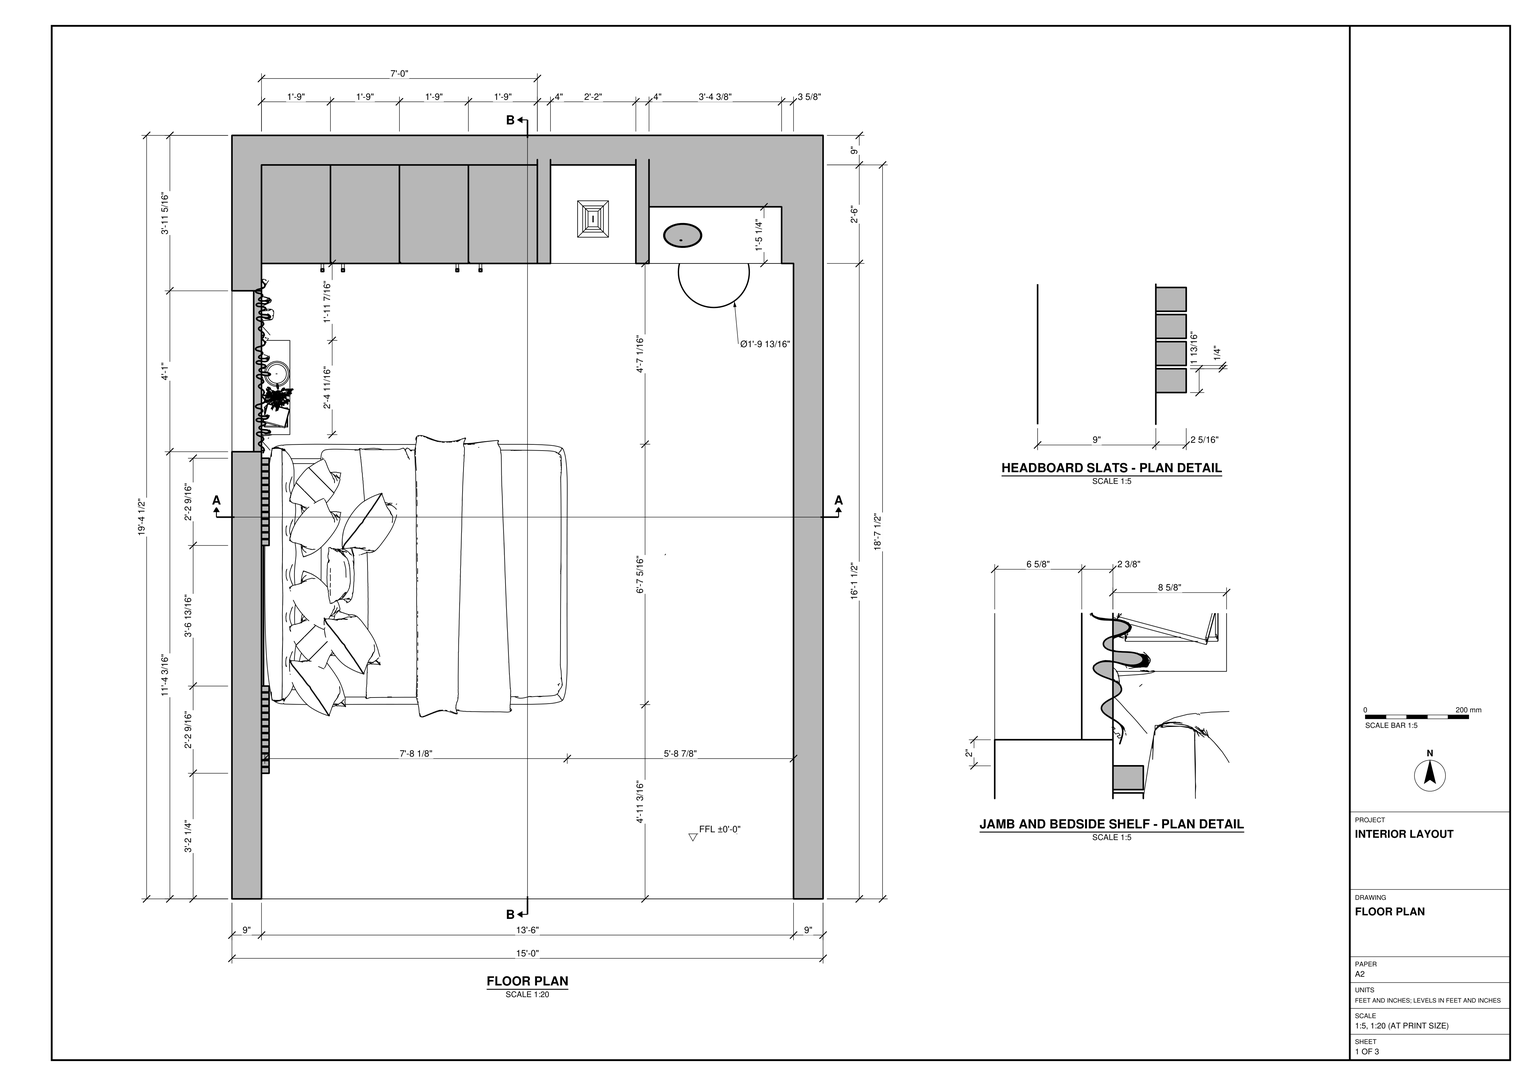
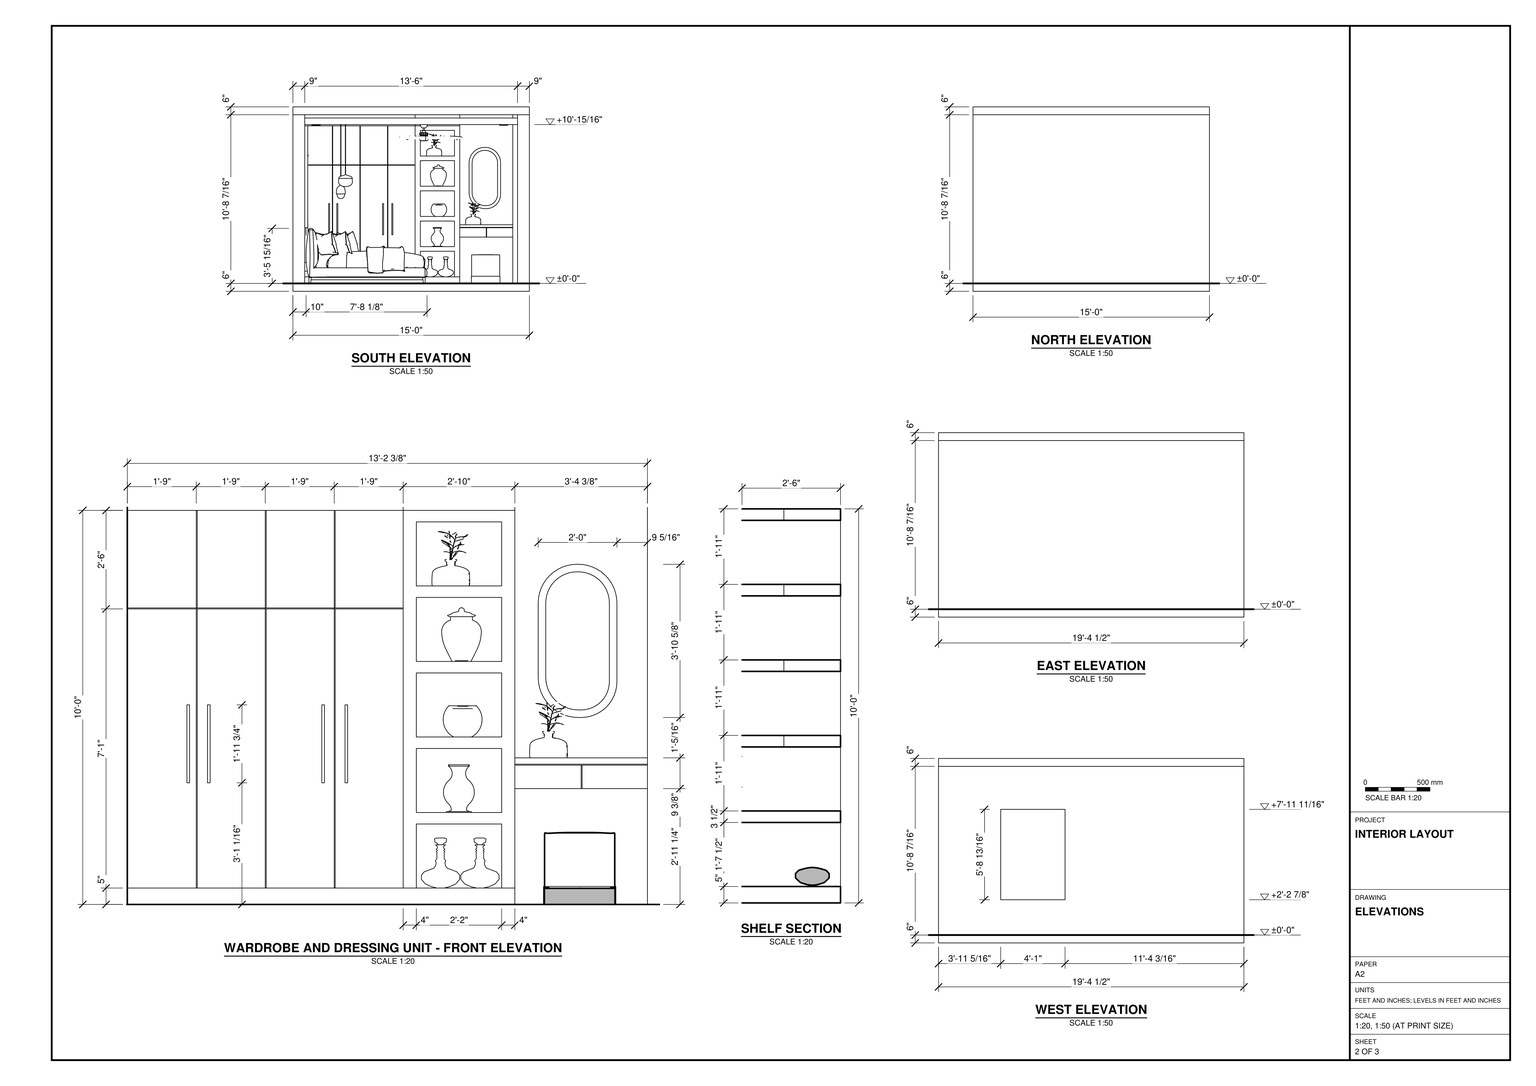
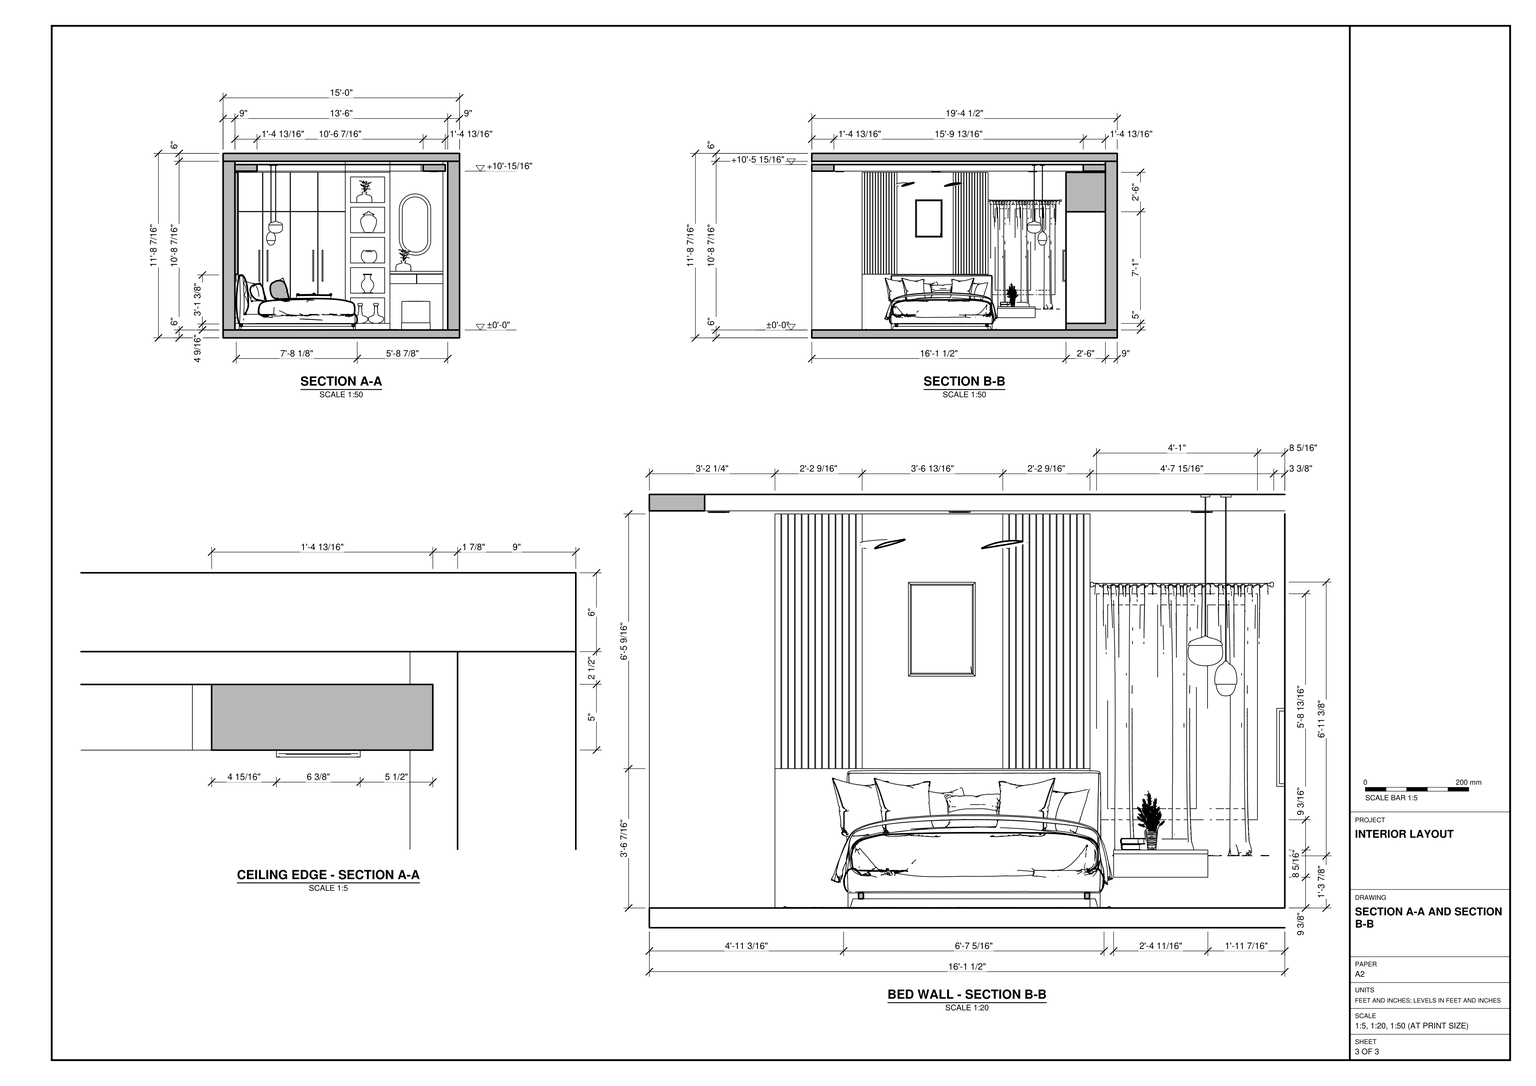
Build the furnished bedroom in SketchUp from task_files/diagram_01.pdf. Work in feet and inches. The overall model is 15'-0" wide, 19'-4 1/2" deep and 11'-8 7/16" high, with the finished floor at ±0'-0". Form the floor and overhead slabs, the stepped ceiling edge and the 9" north, east and west walls. Leave the south side open as drawn and form the window opening in the west wall.

Place the bed with its head against the west wall and its foot toward the clear aisle along the east wall. Use the bed-wall section to set out the headboard, the two fields of vertical slats and the plain panel between them. Fit the low bedside shelf beneath the window. Along the north wall, model the wardrobe with its upper cupboards, the adjoining open display shelves and the dressing counter with drawers, mirror and stool. Use the joinery elevation for the front divisions and the plan for the different depths.

Decor and loose items, including the curtains, cushions, pendant lights, plants and shelf objects, may be any suitable library components. Keep the shell elements and each furniture or joinery piece in separate groups or components, and use components for repeated parts. Save one SketchUp model as output_files/bedroom_with_fitted_storage_and_a_slatted_bed_wall.skp.

# SketchUp Ruby script. Lengths in inches.
U = 1.inch
M = Sketchup.active_model
def pt(a) = Geom::Point3d.new(a.map { |v| v * U })
def face(e, loops, mat)
  f = e.add_face(loops[0].map { |a| pt(a) })
  loops[1..].each { |l| e.add_face(l.map { |a| pt(a) }).erase! }
  f.material = f.back_material = mat if mat
  f
end
# faces: each face lists its corners as indices into pts; further lists are holes
def faces(e, pts, list, mat = nil) = list.each { |f| face(e, (f[0].is_a?(Array) ? f : [f]).map { |l| l.map { |i| pts[i] } }, mat) }
# xy, xz, yz: faces in a plane at the given z, y or x. An outline is a flat list of corners, or four numbers for a rectangle; further outlines are holes
def ring(l) = l.size == 4 ? [[l[0], l[1]], [l[2], l[1]], [l[2], l[3]], [l[0], l[3]]] : l.each_slice(2).to_a
def flat(e, list, mat, &to3) = list.each { |f| face(e, (f[0].is_a?(Array) ? f : [f]).map { |l| ring(l).map { |u, v| to3.(u, v) } }, mat) }
def xy(e, z, list, mat = nil) = flat(e, list, mat) { |x, y| [x, y, z] }
def xz(e, y, list, mat = nil) = flat(e, list, mat) { |x, z| [x, y, z] }
def yz(e, x, list, mat = nil) = flat(e, list, mat) { |y, z| [x, y, z] }
def lines(e, pts, list) = list.each { |a, b| e.add_line(pt(pts[a]), pt(pts[b])) }
# prism: a flat outline (further loops are holes) pulled along v
def prism(e, loops, v, mat = nil)
  f = face(e, loops, mat); d = Geom::Vector3d.new(v.map { |x| x * U })
  f.pushpull(f.normal.samedirection?(d) ? d.length : -d.length)
end
def box(e, o, s, mat = nil) = prism(e, [[o, [o[0] + s[0], o[1], o[2]], [o[0] + s[0], o[1] + s[1], o[2]], [o[0], o[1] + s[1], o[2]]]], [0, 0, s[2]], mat)
def at(x, y, z, deg = 0) = Geom::Transformation.translation(pt([x, y, z])) * Geom::Transformation.rotation(ORIGIN, Z_AXIS, deg.degrees)
def axes(o, x, y, z) = Geom::Transformation.new([*x, 0, *y, 0, *z, 0, *pt(o).to_a, 1])
def part(name) = M.definitions.add(name)
# library, detail: a bought-in or finely detailed component or shape, given as its bounding box
def library(name, o, s) = part(name).tap { |d| box(d.entities, o, s) }
def detail(e, o, s) = box(e.add_group.entities, o, s)
def put(e, d, t, mat = nil) = e.add_instance(d, t).tap { |i| i.material = mat if mat }
def group(e, t, mat = nil) = e.add_group.tap { |g| g.transformation = t; g.material = mat if mat }.entities
root = M.entities
M.materials.add("160").color = [42, 54, 41]
M.materials.add("Generic").color = [133, 143, 95]
M.materials.add("Generic\#1").color = [236, 224, 156]
M.materials.add("Generic\#2").color = [159, 178, 113]
M.materials.add("Generic\#3").color = [244, 241, 241]
M.materials.add("Watercolor Leaves").color = [227, 230, 228]
M.materials.add("[0010_Snow]").color = [255, 250, 250]
M.materials.add("[Color E07]").color = [145, 145, 78]
M.materials.add("[Color M00]").color = [255, 255, 255]
M.materials.add("[Mirror 01]").color = [185, 185, 185]
M.materials.add("[Translucent Glass Gray]").color = [150, 150, 150]
M.materials["[Translucent Glass Gray]"].alpha = 0.22
c1 = library("Throw pillow \#2",[0,0,0],[18.68,14.93,15.72])
c2 = library("Throw pillow",[0,0,0],[20.53,16.77,17.73])
c3 = library("Bed pillow",[0,0,0],[375.21,190.09,258.97])
c4 = library("Throw pillow \#1",[0,0,0],[18.68,14.93,15.72])
c5 = library("wwwwwwww",[-8.24,-7.52,-61.35],[14.91,17.06,61.35])
c6 = library("stone+Jar+4",[7.875,-15.36,0],[26.34,31.07,40.68])
c7 = library("Candle Holder",[-3.9375,-3.9375,0],[7.875,7.875,5.91])
c8 = library("Dried grass arrangement",[0,0,0],[11.54,10.2,23.4375])
c9 = library("Flower_pot 07",[-1.21,-1.21,0],[8.32,8.32,4.71])
c10 = library("00000871-book1",[-1.17,-10.85,-0.02],[14.86,13.34,6.32])
c11 = library("Lidded jar",[0,0,0],[13.42,13.42,18.18])
c12 = library("Plant1",[-0.09,-1.87,0],[3.22,5.78,8.62])
c13 = library("Avation+Styled+Ceiling+Fan_JSB",[-19.77,-29.63,-13.8125],[51.59,58.16,13.8125])
c14 = library("Tlon Light 450 Ceiling 152 006",[-8.86,-8.86,-3.78],[17.72,17.72,3.56])
c15 = part("Group\#1")
xy(c15.entities,0,[[0,0,2.3125,1.8125]])
xy(c15.entities,77.57,[[0,0,2.3125,1.8125]])
xz(c15.entities,0,[[0,0,2.3125,77.57]])
xz(c15.entities,1.8125,[[0,0,2.3125,77.57]])
yz(c15.entities,2.3125,[[0,0,1.8125,77.57]])
c16 = library("mesh-256",[-120.04,-169.59,0.14],[253.19,307.8,1.7])
c17 = library("Group10",[-94.75,-3.97,0],[199.87,106.11,39.4375])
c18 = library("mesh-258",[-96.03,-121.28,21.97],[201.42,163.89,40.48])
c19 = library("mesh-263\#1",[-97.08,-118.58,12.75],[201.41,233.93,94.93])
c20 = library("Group20",[-0.01,-0.01,0.02],[107.76,124.16,6.31])
c21 = library("mesh-264",[-106.11,-80.86,12.52],[217.88,74.95,54.44])
c22 = library("Group\#7",[0,0,0],[20.79,20.79,27.22])
c23 = library("Group\#8",[0,0,0],[86.43,11.96,86.84])
c24 = library("Group8\#1",[-7.8,-7.73,0.125],[15.45,15.45,3.88])
c25 = library("Group19\#1",[-7.66,-7.58,3.61],[15.16,15.16,12.05])
c26 = part("Agrupar\#12")
xy(c26.entities,0,[[0,13.9375,0,31.5,0.51,30.98,0.51,14.45]])
xy(c26.entities,1.0625,[[0.51,14.45,0.51,30.98,0.79,30.71,0.79,14.72]])
xy(c26.entities,1.26,[[0,13.9375,0.79,14.72,0.79,30.71,0,31.5]])
yz(c26.entities,0,[[13.9375,0,31.5,1.26]])
yz(c26.entities,0.51,[[14.45,0,30.98,1.0625]])
yz(c26.entities,0.79,[[14.72,1.0625,30.71,1.26]])
p = [[0.79,14.72,1.26],[0,13.9375,1.26],[0,13.9375,0],[0.51,14.45,0],[0.51,14.45,1.0625],[0.79,14.72,1.0625],
  [0,31.5,1.26],[0.79,30.71,1.26],[0.79,30.71,1.0625],[0.51,30.98,1.0625],[0.51,30.98,0],[0,31.5,0]]
faces(c26.entities,p,[[0,1,2,3,4,5],[6,7,8,9,10,11]])
c27 = part("Agrupar\#31")
xy(c27.entities,0,[[0,6.85,0,31.5,0.51,30.98,0.51,7.36]])
xy(c27.entities,1.0625,[[0.51,7.36,0.51,30.98,0.79,30.71,0.79,7.64]])
xy(c27.entities,1.26,[[0,6.85,0.79,7.64,0.79,30.71,0,31.5]])
yz(c27.entities,0,[[6.85,0,31.5,1.26]])
yz(c27.entities,0.51,[[7.36,0,30.98,1.0625]])
yz(c27.entities,0.79,[[7.64,1.0625,30.71,1.26]])
p = [[0.79,7.64,1.26],[0,6.85,1.26],[0,6.85,0],[0.51,7.36,0],[0.51,7.36,1.0625],[0.79,7.64,1.0625],
  [0,31.5,1.26],[0.79,30.71,1.26],[0.79,30.71,1.0625],[0.51,30.98,1.0625],[0.51,30.98,0],[0,31.5,0]]
faces(c27.entities,p,[[0,1,2,3,4,5],[6,7,8,9,10,11]])
c28 = part("Agrupar\#29")
put(c28.entities,c26,at(0,-13.9375,0),"[Color M00]")
put(c28.entities,c27,at(31.5,0,0,90),"[Color M00]")
put(c28.entities,c26,at(24.65,31.5,0,-180),"[Color M00]")
put(c28.entities,c27,at(-6.85,17.56,0,-90),"[Color M00]")
xy(root,-6,[[0,0,180,232.5]])
xy(root,0,[[0,0,9,0,9,193.5,127,193.5,127,230.625,167.375,230.625,167.375,193.5,171,193.5,171,0,180,0,180,232.5,0,232.5],[9,0,171,0,171,193.5,167.375,193.5,167.375,230.625,127,230.625,127,193.5,9,193.5]])
xy(root,5,[[9,193.5,30,223.5],[30,193.5,30.3,193.8],[30.3,193.5,51,193.5,51,223.5,30,223.5,30,193.8,30.3,193.8],[51,193.5,51.3,193.8],[51.3,193.5,72,193.5,72,223.5,51,223.5,51,193.8,51.3,193.8],
  [72,193.5,72.3,193.8],[72.3,193.5,93,193.5,93,223.5,72,223.5,72,193.8,72.3,193.8],[93,193.5,97,225.125],[97,193.5,123,223.5]])
xy(root,9.35,[[9,141.38,17.65,170.07]])
xy(root,16.48,[[9,141.38,17.65,170.07]])
xy(root,17.66,[[9,141.38,17.65,170.07]])
xy(root,24.5,[[97,193.5,123,223.5],[97,223.5,123,225.125]])
xy(root,26.87,[[0,136.17,9,185.17]])
xy(root,28,[[97,193.5,123,223.5],[97,223.5,123,225.125]])
xy(root,35.28,[[127,193.5,127,230.625,167.375,230.625,167.375,193.5,147.49,193.5,147.49,193.8,147.1875,193.8,147.1875,193.5]])
xy(root,37.86,[[27.15,191.85,27.95,193.5],[33.41,191.85,34.21,193.5],[68.23,191.85,69.02,193.5],[75.29,191.85,76.09,193.5]])
xy(root,42.41,[[127,193.5,147.1875,193.8],[147.49,193.5,167.375,193.8]])
xy(root,42.43,[[9,64.8125,9.625,107.625]])
xy(root,42.71,[[127,193.5,167.375,193.8]])
xy(root,44.65,[[127,193.5,167.375,210.75]])
xy(root,47.5,[[97,193.5,123,223.5],[97,223.5,123,225.125]])
xy(root,51,[[97,193.5,123,223.5],[97,223.5,123,225.125]])
xy(root,56.93,[[146.34,207.1875,147.15,210.75]])
xy(root,59.24,[[146.34,207.1875,147.15,208.625]])
xy(root,60.79,[[27.95,191.03,27.95,193.5,27.15,193.5,27.15,191.04],[34.21,191.03,34.21,193.5,33.41,193.5,33.41,191.04],[69.02,191.03,69.02,193.5,68.23,193.5,68.23,191.04],[76.09,191.03,76.09,193.5,75.29,193.5,75.29,191.04]])
xy(root,70.5,[[97,193.5,123,223.5],[97,223.5,123,225.125]])
xy(root,74,[[97,193.5,123,223.5],[97,223.5,123,225.125]])
xy(root,90,[[9,193.5,30,193.8],[30.3,193.5,51,193.8],[51.3,193.5,72,193.8],[72.3,193.5,93,193.8],[9,193.8,30,223.5],
  [30,193.8,51,223.5],[51,193.8,72,223.5],[72,193.8,93,223.5]])
xy(root,90.3,[[9,193.5,30,193.8],[30.3,193.5,51,193.8],[51.3,193.5,72,193.8],[72.3,193.5,93,193.8]])
xy(root,93.5,[[97,193.5,123,223.5],[97,223.5,123,225.125]])
xy(root,95.68,[[0,136.17,9,185.17]])
xy(root,97,[[97,193.5,123,223.5],[97,223.5,123,225.125]])
xy(root,116.5,[[97,193.5,123,223.5],[97,223.5,123,225.125]])
xy(root,120,[[9,64.8125,9.625,107.625],[9,193.5,30,223.5],[30.3,193.5,51,193.5,51,223.5,30,223.5,30,193.8,30.3,193.8],[51.3,193.5,72,193.5,72,223.5,51,223.5,51,193.8,51.3,193.8],[72.3,193.5,93,193.5,93,223.5,72,223.5,72,193.8,72.3,193.8],
  [93,193.5,127,225.125]])
xy(root,120.9375,[[[9,0,9,223.5,167.375,223.5,171,0],[25.84,16.84,153.89,16.84,150.8125,206.66,25.84,206.66]]],"Generic\#3")
xy(root,125.9375,[[[9,0,171,0,167.375,223.5,9,223.5],[25.84,16.84,25.84,206.66,150.8125,206.66,153.89,16.84]]])
xy(root,125.9375,[[25.84,16.84,25.84,206.66,150.8125,206.66,153.89,16.84]],"Generic\#3")
xy(root,128.4375,[[0,0,9,232.5],[9,0,9,223.5,93,223.5,93,225.125,127,225.125,127,210.75,167.375,210.75,167.375,193.5,171,193.5,171,0],[171,0,180,0,180,232.5,127,232.5,127,210.75,167.375,210.75,167.375,193.5,171,193.5],[9,223.5,93,232.5],[93,225.125,127,232.5]])
xy(root,134.4375,[[0,0,180,232.5]])
xz(root,0,[[0,-6,180,0],[0,0,9,128.4375],[171,0,180,128.4375],[9,120.9375,171,125.9375],[0,128.4375,180,134.4375]])
xz(root,16.84,[[25.84,120.9375,153.89,125.9375]])
xz(root,64.8125,[[9,42.43,9.625,120]])
xz(root,107.625,[[9,42.43,9.625,120]])
xz(root,136.17,[[0,26.87,9,95.68]])
xz(root,141.38,[[9,9.35,17.65,16.48],[9,16.48,17.65,17.66]])
xz(root,170.07,[[9,9.35,17.65,16.48],[9,16.48,17.65,17.66]])
xz(root,185.17,[[0,26.87,9,95.68]])
xz(root,191.85,[[27.15,37.86,27.15,59.97,27.95,59.98,27.95,37.86],[33.41,37.86,33.41,59.97,34.21,59.98,34.21,37.86],[68.23,37.86,68.23,59.97,69.02,59.98,69.02,37.86],[75.29,37.86,75.29,59.97,76.09,59.98,76.09,37.86]])
xz(root,193.5,[[9,0,127,5],[167.375,0,171,128.4375],[[9,5,30,90],[27.15,59.97,27.15,60.79,27.95,60.79,27.95,59.98],[27.95,37.04,27.15,37.05,27.15,37.86,27.95,37.86]],[[30.3,5,51,90],[33.41,59.97,33.41,60.79,34.21,60.79,34.21,59.98],[34.21,37.04,33.41,37.05,33.41,37.86,34.21,37.86]],[[51.3,5,72,90],[68.23,59.97,68.23,60.79,69.02,60.79,69.02,59.98],[69.02,37.04,68.23,37.05,68.23,37.86,69.02,37.86]],
  [[72.3,5,93,90],[75.29,59.97,75.29,60.79,76.09,60.79,76.09,59.98],[76.09,37.04,75.29,37.05,75.29,37.86,76.09,37.86]],[[93,5,97,5,97,24.5,123,24.5,123,5,127,5,127,120,93,120],[97,51,123,70.5],[97,97,123,116.5],[97,74,123,93.5],[97,28,123,47.5]],[127,35.28,147.1875,42.41],[147.49,35.28,167.375,42.41],[127,42.71,167.375,44.65],
  [27.15,59.97,27.15,60.79,27.95,60.79,27.95,59.98],[33.41,59.97,33.41,60.79,34.21,60.79,34.21,59.98],[68.23,59.97,68.23,60.79,69.02,60.79,69.02,59.98],[75.29,59.97,75.29,60.79,76.09,60.79,76.09,59.98],[9,90.3,30,120],
  [30.3,90.3,51,120],[51.3,90.3,72,120],[72.3,90.3,93,120]])
xz(root,193.8,[[30,5,30.3,90],[51,5,51.3,90],[72,5,72.3,90],[147.1875,35.28,147.49,42.41],[127,42.41,167.375,42.71],
  [9,90,30,90.3],[30,90,51,90.3],[51,90,72,90.3],[72,90,93,90.3],[30,90.3,30.3,120],
  [51,90.3,51.3,120],[72,90.3,72.3,120]])
xz(root,206.66,[[25.84,120.9375,93,125.9375],[93,120.9375,127,125.9375]])
xz(root,206.66,[[127,120.9375,150.8125,125.9375]],"Generic\#3")
xz(root,207.1875,[[[146.34,56.93,147.15,56.93,148.58,57.03,149.98,57.31,151.34,57.77,152.62,58.4,153.81,59.19,154.88,60.14,155.83,61.21,156.62,62.4,157.25,63.69,157.71,65.04,157.99,66.44,158.09,67.87,158.09,91.79,157.98,93.375,157.66,94.92,157.14,96.42,156.43,97.83,155.53,99.13,154.47,100.3,153.26,101.32,151.92,102.17,150.48,102.83,148.97,103.3,147.41,103.55,145.91,103.6,144.37,103.5,142.86,103.2,141.4,102.7,140.01,102.02,138.73,101.16,137.57,100.14,136.55,98.98,135.69,97.7,135.01,96.3125,134.51,94.85,134.21,93.34,134.11,91.79,134.11,69.17,134.21,67.57,134.53,66,135.04,64.49,135.75,63.05,136.64,61.72,137.69,60.52,138.89,59.46,140.23,58.57,141.66,57.87,143.18,57.35,144.74,57.04],[146.34,59.24,145.05,59.32,143.77,59.57,142.54,59.99,141.375,60.57,140.3,61.29,139.32,62.14,138.46,63.12,137.74,64.2,137.17,65.37,136.75,66.6,136.5,67.87,136.41,69.17,136.41,91.79,136.49,93.04,136.73,94.25,137.13,95.43,137.68,96.55,138.375,97.58,139.19,98.51,140.13,99.33,141.16,100.02,142.28,100.57,143.45,100.97,144.67,101.22,145.91,101.3,147.1875,101.26,148.44,101.05,149.66,100.68,150.82,100.15,151.9,99.47,152.87,98.65,153.73,97.7,154.45,96.65,155.03,95.52,155.45,94.3125,155.7,93.07,155.79,91.79,155.79,67.87,155.71,66.74,155.49,65.64,155.13,64.57,154.63,63.55,154,62.61,153.26,61.76,152.41,61.02,151.47,60.39,150.45,59.89,149.39,59.53,148.28,59.31,147.15,59.24]]])
xz(root,208.625,[[146.34,59.24,147.15,59.24,148.28,59.31,149.39,59.53,150.45,59.89,151.47,60.39,152.41,61.02,153.26,61.76,154,62.61,154.63,63.55,155.13,64.57,155.49,65.64,155.71,66.74,155.79,67.87,155.79,91.79,155.7,93.07,155.45,94.3125,155.03,95.52,154.45,96.65,153.73,97.7,152.87,98.65,151.9,99.47,150.82,100.15,149.66,100.68,148.44,101.05,147.1875,101.26,145.91,101.3,144.67,101.22,143.45,100.97,142.28,100.57,141.16,100.02,140.13,99.33,139.19,98.51,138.375,97.58,137.68,96.55,137.13,95.43,136.73,94.25,136.49,93.04,136.41,91.79,136.41,69.17,136.5,67.87,136.75,66.6,137.17,65.37,137.74,64.2,138.46,63.12,139.32,62.14,140.3,61.29,141.375,60.57,142.54,59.99,143.77,59.57,145.05,59.32]],"[Mirror 01]")
xz(root,210.75,[[[127,44.65,167.375,128.4375],[146.34,56.93,144.74,57.04,143.18,57.35,141.66,57.87,140.23,58.57,138.89,59.46,137.69,60.52,136.64,61.72,135.75,63.05,135.04,64.49,134.53,66,134.21,67.57,134.11,69.17,134.11,91.79,134.21,93.34,134.51,94.85,135.01,96.3125,135.69,97.7,136.55,98.98,137.57,100.14,138.73,101.16,140.01,102.02,141.4,102.7,142.86,103.2,144.37,103.5,145.91,103.6,147.41,103.55,148.97,103.3,150.48,102.83,151.92,102.17,153.26,101.32,154.47,100.3,155.53,99.13,156.43,97.83,157.14,96.42,157.66,94.92,157.98,93.375,158.09,91.79,158.09,67.87,157.99,66.44,157.71,65.04,157.25,63.69,156.62,62.4,155.83,61.21,154.88,60.14,153.81,59.19,152.62,58.4,151.34,57.77,149.98,57.31,148.58,57.03,147.15,56.93]]])
xz(root,223.5,[[9,5,30,90],[30,5,51,90],[51,5,72,90],[72,5,93,90],[97,5,123,24.5],
  [97,28,123,47.5],[97,51,123,70.5],[97,74,123,93.5],[9,90,30,120],[30,90,51,120],
  [51,90,72,120],[72,90,93,120],[97,97,123,116.5],[9,120,93,120.9375],[9,120.9375,93,125.9375],
  [93,120.9375,127,125.9375],[127,120.9375,163.75,125.9375],[163.75,120.9375,167.375,125.9375],[9,125.9375,93,128.4375]])
xz(root,225.125,[[93,120,127,128.4375]])
xz(root,230.625,[[127,0,167.375,35.28]])
xz(root,232.5,[[0,-6,180,0],[0,0,180,128.4375],[0,128.4375,180,134.4375]])
yz(root,0,[[0,-6,232.5,0],[[0,0,232.5,128.4375],[136.17,26.87,185.17,95.68]],[0,128.4375,232.5,134.4375]])
yz(root,9,[[[0,0,38.25,0,38.25,42.43,64.8125,42.43,64.8125,120,107.625,120,107.625,42.43,134.1875,42.43,134.1875,0,193.5,0,193.5,90,193.8,90,193.8,90.3,193.5,90.3,193.5,120,223.5,120,223.5,120.9375,0,120.9375],[136.17,26.87,185.17,95.68],[141.38,9.35,170.07,17.66]],[38.25,0,134.1875,42.43],[193.5,5,223.5,90],[141.38,9.35,170.07,16.48],[141.38,16.48,170.07,17.66],
  [64.8125,42.43,107.625,120],[193.8,90,223.5,90,223.5,120,193.5,120,193.5,90.3,193.8,90.3],[0,120.9375,223.5,125.9375],[0,125.9375,223.5,128.4375]])
yz(root,9.625,[[64.8125,42.43,107.625,120]],"Generic\#2")
yz(root,17.65,[[141.38,9.35,170.07,16.48],[141.38,16.48,170.07,17.66]])
yz(root,25.84,[[16.84,120.9375,206.66,125.9375]],"Generic\#3")
yz(root,27.15,[[191.04,37.05,191.04,60.79,193.5,60.79,193.5,59.97,191.85,59.97,191.85,37.86,193.5,37.86,193.5,37.05]])
yz(root,27.95,[[191.03,37.04,193.5,37.04,193.5,37.86,191.85,37.86,191.85,59.98,193.5,59.98,193.5,60.79,191.03,60.79]])
yz(root,30,[[193.5,5,193.8,90],[193.8,5,223.5,90],[193.8,90,223.5,120],[193.5,90.3,193.8,120]])
yz(root,30.3,[[193.5,5,193.8,90],[193.5,90.3,193.8,120]])
yz(root,33.41,[[191.04,37.05,191.04,60.79,193.5,60.79,193.5,59.97,191.85,59.97,191.85,37.86,193.5,37.86,193.5,37.05]])
yz(root,34.21,[[191.03,37.04,193.5,37.04,193.5,37.86,191.85,37.86,191.85,59.98,193.5,59.98,193.5,60.79,191.03,60.79]])
yz(root,51,[[193.5,5,193.8,90],[193.8,5,223.5,90],[193.8,90,223.5,120],[193.5,90.3,193.8,120]])
yz(root,51.3,[[193.5,5,193.8,90],[193.5,90.3,193.8,120]])
yz(root,68.23,[[191.04,37.05,191.04,60.79,193.5,60.79,193.5,59.97,191.85,59.97,191.85,37.86,193.5,37.86,193.5,37.05]])
yz(root,69.02,[[191.03,37.04,193.5,37.04,193.5,37.86,191.85,37.86,191.85,59.98,193.5,59.98,193.5,60.79,191.03,60.79]])
yz(root,72,[[193.5,5,193.8,90],[193.8,5,223.5,90],[193.8,90,223.5,120],[193.5,90.3,193.8,120]])
yz(root,72.3,[[193.5,5,193.8,90],[193.5,90.3,193.8,120]])
yz(root,75.29,[[191.04,37.05,191.04,60.79,193.5,60.79,193.5,59.97,191.85,59.97,191.85,37.86,193.5,37.86,193.5,37.05]])
yz(root,76.09,[[191.03,37.04,193.5,37.04,193.5,37.86,191.85,37.86,191.85,59.98,193.5,59.98,193.5,60.79,191.03,60.79]])
yz(root,93,[[193.5,5,223.5,90],[223.5,5,225.125,90],[193.5,90,193.8,90.3],[193.8,90,193.8,90.3,193.5,90.3,193.5,120,223.5,120,223.5,90],[223.5,90,225.125,120],
  [223.5,120,225.125,128.4375]])
yz(root,97,[[193.5,5,223.5,24.5],[223.5,5,225.125,24.5],[193.5,28,223.5,47.5],[223.5,28,225.125,47.5],[193.5,51,223.5,70.5],
  [223.5,51,225.125,70.5],[193.5,74,223.5,93.5],[223.5,74,225.125,93.5],[193.5,97,223.5,116.5],[223.5,97,225.125,116.5]])
yz(root,123,[[193.5,5,223.5,24.5],[223.5,5,225.125,24.5],[193.5,28,223.5,47.5],[223.5,28,225.125,47.5],[193.5,51,223.5,70.5],
  [223.5,51,225.125,70.5],[193.5,74,223.5,93.5],[223.5,74,225.125,93.5],[193.5,97,223.5,116.5],[223.5,97,225.125,116.5]])
yz(root,127,[[193.5,0,230.625,35.28],[193.5,35.28,225.125,35.28,225.125,44.65,193.5,44.65,193.5,42.71,193.8,42.71,193.8,42.41,193.5,42.41],[193.5,42.41,193.8,42.71],[193.5,44.65,210.75,120],[210.75,44.65,225.125,120],
  [210.75,120,225.125,128.4375]])
yz(root,134.11,[[207.1875,69.17,210.75,91.79]])
yz(root,136.41,[[207.1875,69.17,208.625,91.79]])
yz(root,147.1875,[[193.5,35.28,193.8,42.41]])
yz(root,147.49,[[193.5,35.28,193.8,42.41]])
yz(root,155.79,[[207.1875,67.87,208.625,91.79]])
yz(root,158.09,[[207.1875,67.87,210.75,91.79]])
yz(root,167.375,[[193.5,0,230.625,35.28],[193.5,42.41,193.8,42.71],[193.5,44.65,210.75,128.4375]])
yz(root,171,[[0,0,193.5,128.4375]])
yz(root,180,[[0,-6,232.5,0],[0,0,232.5,128.4375],[0,128.4375,232.5,134.4375]])
p = [[27.95,191.03,60.79],[27.15,191.04,60.79],[27.15,191.04,37.05],[27.95,191.03,37.04],[27.15,193.5,37.05],[27.95,193.5,37.04],
  [34.21,191.03,60.79],[33.41,191.04,60.79],[33.41,191.04,37.05],[34.21,191.03,37.04],[33.41,193.5,37.05],[34.21,193.5,37.04],
  [69.02,191.03,60.79],[68.23,191.04,60.79],[68.23,191.04,37.05],[69.02,191.03,37.04],[68.23,193.5,37.05],[69.02,193.5,37.04],
  [76.09,191.03,60.79],[75.29,191.04,60.79],[75.29,191.04,37.05],[76.09,191.03,37.04],[75.29,193.5,37.05],[76.09,193.5,37.04],
  [144.74,210.75,57.04],[146.34,210.75,56.93],[146.34,207.1875,56.93],[144.74,207.1875,57.04],[147.15,210.75,56.93],[148.58,210.75,57.03],
  [148.58,207.1875,57.03],[147.15,207.1875,56.93],[143.18,210.75,57.35],[143.18,207.1875,57.35],[149.98,210.75,57.31],[149.98,207.1875,57.31],
  [151.34,210.75,57.77],[151.34,207.1875,57.77],[141.66,210.75,57.87],[141.66,207.1875,57.87],[152.62,210.75,58.4],[152.62,207.1875,58.4],
  [140.23,210.75,58.57],[140.23,207.1875,58.57],[153.81,210.75,59.19],[153.81,207.1875,59.19],[138.89,210.75,59.46],[138.89,207.1875,59.46],
  [146.34,208.625,59.24],[145.05,208.625,59.32],[145.05,207.1875,59.32],[146.34,207.1875,59.24],[148.28,208.625,59.31],[147.15,208.625,59.24],
  [147.15,207.1875,59.24],[148.28,207.1875,59.31],[154.88,210.75,60.14],[154.88,207.1875,60.14],[143.77,208.625,59.57],[143.77,207.1875,59.57],
  [149.39,208.625,59.53],[149.39,207.1875,59.53],[137.69,210.75,60.52],[137.69,207.1875,60.52],[150.45,208.625,59.89],[150.45,207.1875,59.89],
  [142.54,208.625,59.99],[142.54,207.1875,59.99],[151.47,208.625,60.39],[151.47,207.1875,60.39],[27.15,193.5,59.97],[27.95,193.5,59.98],
  [27.95,191.85,59.98],[27.15,191.85,59.97],[33.41,193.5,59.97],[34.21,193.5,59.98],[34.21,191.85,59.98],[33.41,191.85,59.97],
  [68.23,193.5,59.97],[69.02,193.5,59.98],[69.02,191.85,59.98],[68.23,191.85,59.97],[75.29,193.5,59.97],[76.09,193.5,59.98],
  [76.09,191.85,59.98],[75.29,191.85,59.97],[141.375,208.625,60.57],[141.375,207.1875,60.57],[155.83,210.75,61.21],[155.83,207.1875,61.21],
  [152.41,208.625,61.02],[152.41,207.1875,61.02],[136.64,210.75,61.72],[136.64,207.1875,61.72],[140.3,208.625,61.29],[140.3,207.1875,61.29],
  [153.26,208.625,61.76],[153.26,207.1875,61.76],[156.62,210.75,62.4],[156.62,207.1875,62.4],[139.32,208.625,62.14],[139.32,207.1875,62.14],
  [135.75,210.75,63.05],[135.75,207.1875,63.05],[154,208.625,62.61],[154,207.1875,62.61],[138.46,208.625,63.12],[138.46,207.1875,63.12],
  [157.25,210.75,63.69],[157.25,207.1875,63.69],[154.63,208.625,63.55],[154.63,207.1875,63.55],[135.04,210.75,64.49],[135.04,207.1875,64.49],
  [137.74,208.625,64.2],[137.74,207.1875,64.2],[155.13,208.625,64.57],[155.13,207.1875,64.57],[157.71,210.75,65.04],[157.71,207.1875,65.04],
  [137.17,208.625,65.37],[137.17,207.1875,65.37],[134.53,210.75,66],[134.53,207.1875,66],[155.49,208.625,65.64],[155.49,207.1875,65.64],
  [157.99,210.75,66.44],[157.99,207.1875,66.44],[136.75,208.625,66.6],[136.75,207.1875,66.6],[155.71,208.625,66.74],[155.71,207.1875,66.74],
  [134.21,210.75,67.57],[134.21,207.1875,67.57],[158.09,210.75,67.87],[158.09,207.1875,67.87],[136.5,208.625,67.87],[136.5,207.1875,67.87],
  [155.79,208.625,67.87],[155.79,207.1875,67.87],[134.11,210.75,69.17],[134.11,207.1875,69.17],[136.41,208.625,69.17],[136.41,207.1875,69.17],
  [134.21,210.75,93.34],[134.11,210.75,91.79],[134.11,207.1875,91.79],[134.21,207.1875,93.34],[136.41,208.625,91.79],[136.49,208.625,93.04],
  [136.49,207.1875,93.04],[136.41,207.1875,91.79],[155.7,208.625,93.07],[155.79,208.625,91.79],[155.79,207.1875,91.79],[155.7,207.1875,93.07],
  [158.09,210.75,91.79],[157.98,210.75,93.375],[157.98,207.1875,93.375],[158.09,207.1875,91.79],[136.73,208.625,94.25],[136.73,207.1875,94.25],
  [155.45,208.625,94.3125],[155.45,207.1875,94.3125],[134.51,210.75,94.85],[134.51,207.1875,94.85],[157.66,210.75,94.92],[157.66,207.1875,94.92],
  [137.13,208.625,95.43],[137.13,207.1875,95.43],[155.03,208.625,95.52],[155.03,207.1875,95.52],[135.01,210.75,96.3125],[135.01,207.1875,96.3125],
  [157.14,210.75,96.42],[157.14,207.1875,96.42],[137.68,208.625,96.55],[137.68,207.1875,96.55],[154.45,208.625,96.65],[154.45,207.1875,96.65],
  [135.69,210.75,97.7],[135.69,207.1875,97.7],[156.43,210.75,97.83],[156.43,207.1875,97.83],[138.375,208.625,97.58],[138.375,207.1875,97.58],
  [153.73,208.625,97.7],[153.73,207.1875,97.7],[139.19,208.625,98.51],[139.19,207.1875,98.51],[136.55,210.75,98.98],[136.55,207.1875,98.98],
  [152.87,208.625,98.65],[152.87,207.1875,98.65],[155.53,210.75,99.13],[155.53,207.1875,99.13],[140.13,208.625,99.33],[140.13,207.1875,99.33],
  [151.9,208.625,99.47],[151.9,207.1875,99.47],[137.57,210.75,100.14],[137.57,207.1875,100.14],[154.47,210.75,100.3],[154.47,207.1875,100.3],
  [141.16,208.625,100.02],[141.16,207.1875,100.02],[150.82,208.625,100.15],[150.82,207.1875,100.15],[142.28,208.625,100.57],[142.28,207.1875,100.57],
  [138.73,210.75,101.16],[138.73,207.1875,101.16],[149.66,208.625,100.68],[149.66,207.1875,100.68],[153.26,210.75,101.32],[153.26,207.1875,101.32],
  [143.45,208.625,100.97],[143.45,207.1875,100.97],[148.44,208.625,101.05],[148.44,207.1875,101.05],[144.67,208.625,101.22],[144.67,207.1875,101.22],
  [147.1875,208.625,101.26],[147.1875,207.1875,101.26],[140.01,210.75,102.02],[140.01,207.1875,102.02],[145.91,208.625,101.3],[145.91,207.1875,101.3],
  [151.92,210.75,102.17],[151.92,207.1875,102.17],[141.4,210.75,102.7],[141.4,207.1875,102.7],[150.48,210.75,102.83],[150.48,207.1875,102.83],
  [142.86,210.75,103.2],[142.86,207.1875,103.2],[148.97,210.75,103.3],[148.97,207.1875,103.3],[144.37,210.75,103.5],[144.37,207.1875,103.5],
  [147.41,210.75,103.55],[147.41,207.1875,103.55],[145.91,210.75,103.6],[145.91,207.1875,103.6],[167.375,223.5,125.9375],[171,0,125.9375],
  [171,0,120.9375],[167.375,223.5,120.9375],[153.89,16.84,125.9375],[150.8125,206.66,125.9375],[150.8125,206.66,120.9375],[153.89,16.84,120.9375],
  [27.625,193.5,60.45],[27.625,191.375,60.45],[27.625,191.375,37.39],[27.625,193.5,37.39],[33.89,193.5,60.45],[33.89,191.375,60.45],
  [33.89,191.375,37.39],[33.89,193.5,37.39],[68.7,191.375,37.39],[68.7,193.5,37.39],[68.7,193.5,60.45],[68.7,191.375,60.45],
  [75.76,191.375,37.39],[75.76,193.5,37.39],[75.76,193.5,60.45],[75.76,191.375,60.45]]
faces(root,p,[[0,1,2,3],[3,2,4,5],[6,7,8,9],[9,8,10,11],[12,13,14,15],[15,14,16,17],[18,19,20,21],[21,20,22,23],
  [24,25,26,27],[28,29,30,31],[32,24,27,33],[29,34,35,30],[34,36,37,35],[38,32,33,39],[36,40,41,37],[42,38,39,43],
  [40,44,45,41],[46,42,43,47],[48,49,50,51],[52,53,54,55],[44,56,57,45],[49,58,59,50],[60,52,55,61],[62,46,47,63],
  [64,60,61,65],[58,66,67,59],[68,64,65,69],[70,71,72,73],[74,75,76,77],[78,79,80,81],[82,83,84,85],[66,86,87,67],
  [56,88,89,57],[90,68,69,91],[92,62,63,93],[86,94,95,87],[96,90,91,97],[88,98,99,89],[94,100,101,95],[102,92,93,103],
  [104,96,97,105],[100,106,107,101],[98,108,109,99],[110,104,105,111],[112,102,103,113],[106,114,115,107],[116,110,111,117],[108,118,119,109],
  [114,120,121,115],[122,112,113,123],[124,116,117,125],[118,126,127,119],[120,128,129,121],[130,124,125,131],[132,122,123,133],[126,134,135,127],
  [128,136,137,129],[138,130,131,139],[140,132,133,141],[136,142,143,137],[144,145,146,147],[148,149,150,151],[152,153,154,155],[156,157,158,159],
  [149,160,161,150],[162,152,155,163],[164,144,147,165],[157,166,167,158],[160,168,169,161],[170,162,163,171],[172,164,165,173],[166,174,175,167],
  [168,176,177,169],[178,170,171,179],[180,172,173,181],[174,182,183,175],[176,184,185,177],[186,178,179,187],[184,188,189,185],[190,180,181,191],
  [192,186,187,193],[182,194,195,183],[188,196,197,189],[198,192,193,199],[200,190,191,201],[194,202,203,195],[196,204,205,197],[206,198,199,207],
  [204,208,209,205],[210,200,201,211],[212,206,207,213],[202,214,215,203],[208,216,217,209],[218,212,213,219],[216,220,221,217],[222,218,219,223],
  [224,210,211,225],[220,226,227,221],[226,222,223,227],[214,228,229,215],[230,224,225,231],[228,232,233,229],[234,230,231,235],[232,236,237,233],
  [238,234,235,239],[236,240,241,237],[242,238,239,243],[240,242,243,241],[244,245,246,247]])
faces(root,p,[[248,249,250,251]],"Generic\#3")
lines(root,p,[[252,253],[253,254],[254,255],[256,257],[258,259],[257,258],[260,261],[262,263],[263,260],[264,265],[266,267],[267,264]])
put(root,c1,axes([33.27,122.53,22.08],[-0.02054,-0.99859,-0.04897],[-0.9991,0.02233,-0.03615],[-0.03719,-0.04819,0.99815]))
put(root,c2,axes([34.72,55.09,21.98],[-0.01345,0.99918,-0.03811],[-0.99977,-0.01407,-0.01614],[-0.01667,0.03789,0.99914]))
put(root,c3,axes([38.15,90.46,24.49],[-0.00366,0.04597,0],[-0.04557,-0.00444,0],[0,0,0.03952]))
put(root,c4,axes([33.27,134.53,22.08],[-0.02054,-0.99859,-0.04897],[-0.9991,0.02233,-0.03615],[-0.03719,-0.04819,0.99815]))
put(root,c2,axes([50.76,124.17,21.98],[-0.01345,-0.99918,-0.03811],[-0.99977,0.01407,-0.01614],[-0.01667,-0.03789,0.99914]))
put(root,c1,axes([33.27,81.48,22.08],[-0.02054,0.99859,-0.04897],[-0.9991,-0.02233,-0.03615],[-0.03719,0.04819,0.99815]))
put(root,c4,axes([33.27,69.48,22.08],[-0.02054,0.99859,-0.04897],[-0.9991,-0.02233,-0.03615],[-0.03719,0.04819,0.99815]))
put(root,c2,axes([45.26,67.8125,21.94],[-0.01345,0.99918,-0.03811],[-0.99977,-0.01407,-0.01614],[-0.01667,0.03789,0.99914]))
put(root,c5,at(40.8,169.38,125.9375))
put(root,c6,axes([102.44,206.97,28],[0.3572,0,0],[0,0.3572,0],[0,0,0.3572]))
put(root,c7,at(13.71,159.89,17.66))
put(root,c8,axes([9.25,148.52,16.48],[0.82,0,0],[0,0.82,0],[0,0,0.82]))
put(root,c9,axes([105.15,200.65,51],[2.01661,0,0],[0,2.01661,0],[0,0,2.01661]))
put(root,c10,axes([9.94,149.52,17.68],[0.5628,0,0],[0,0.5628,0],[0,0,0.5628]))
put(root,c11,axes([104.72,196.6875,74],[0.9,0,0],[0,0.9,0],[0,0,0.9]))
put(root,c12,axes([101.75,202.93,97],[3.78896,0,0],[0,2.3572,0],[0,0,2.3572]))
put(root,c12,axes([131.5,197.9,44.65],[3.78896,0,0],[0,2.3572,0],[0,0,2.3572]))
put(root,c13,at(99.65,87.625,122.3125))
put(root,c14,axes([160.4,94.48,121.77],[0.36,0,0],[0,0.36,0],[0,0,0.36]))
put(root,c14,axes([160.4,168.23,121.77],[0.36,0,0],[0,0.36,0],[0,0,0.36]))
put(root,c14,axes([160.4,21.11,121.77],[0.36,0,0],[0,0.36,0],[0,0,0.36]))
put(root,c14,axes([17.59,94.48,121.77],[0.36,0,0],[0,0.36,0],[0,0,0.36]))
put(root,c14,axes([17.59,168.23,121.77],[0.36,0,0],[0,0.36,0],[0,0,0.36]))
put(root,c14,axes([17.59,21.11,121.77],[0.36,0,0],[0,0.36,0],[0,0,0.36]))
put(root,c15,at(9,38.25,42.43),"Generic")
put(root,c15,at(9,40.3125,42.43),"Generic")
put(root,c15,at(9,42.375,42.43),"Generic")
put(root,c15,at(9,44.4375,42.43),"Generic")
put(root,c15,at(9,46.5,42.43),"Generic")
put(root,c15,at(9,48.5625,42.43),"Generic")
put(root,c15,at(9,50.625,42.43),"Generic")
put(root,c15,at(9,52.6875,42.43),"Generic")
put(root,c15,at(9,54.75,42.43),"Generic")
put(root,c15,at(9,56.8125,42.43),"Generic")
put(root,c15,at(9,58.875,42.43),"Generic")
put(root,c15,at(9,60.9375,42.43),"Generic")
put(root,c15,at(9,63,42.43),"Generic")
put(root,c15,at(9,107.625,42.43),"Generic")
put(root,c15,at(9,113.8125,42.43),"Generic")
put(root,c15,at(9,132.375,42.43),"Generic")
put(root,c15,at(9,109.6875,42.43),"Generic")
put(root,c15,at(9,124.125,42.43),"Generic")
put(root,c15,at(9,130.3125,42.43),"Generic")
put(root,c15,at(9,120,42.43),"Generic")
put(root,c15,at(9,117.9375,42.43),"Generic")
put(root,c15,at(9,126.1875,42.43),"Generic")
put(root,c15,at(9,111.75,42.43),"Generic")
put(root,c15,at(9,122.0625,42.43),"Generic")
put(root,c15,at(9,128.25,42.43),"Generic")
put(root,c15,at(9,115.875,42.43),"Generic")
g1 = group(root,at(6.625,136.17,26.87))
xy(g1,0,[[0,0,2.375,49]])
xy(g1,68.8125,[[0,0,2.375,49]],"[0010_Snow]")
xz(g1,0,[[0,0,2.375,68.8125]],"[0010_Snow]")
xz(g1,49,[[0,0,2.375,68.8125]])
yz(g1,0,[[0,0,49,68.8125]],"[Translucent Glass Gray]")
yz(g1,2.375,[[[0,0,49,68.8125],[33.79,3.38,45.62,65.43],[3.38,3.38,15.21,65.43],[18.59,3.38,30.41,65.43]]],"[0010_Snow]")
yz(g1,2.375,[[3.38,3.38,15.21,65.43],[18.59,3.38,30.41,65.43],[33.79,3.38,45.62,65.43]],"[Translucent Glass Gray]")
g2 = group(root,at(65.43,88.08,-0.02))
put(g2,c16,axes([0,0,0],[0,0.3937,0],[-0.3937,0,0],[0,0,0.3937]))
put(root,c17,axes([64.18,97.38,9.2],[0,0.37903,0],[-0.37903,0,0],[0,0,0.37903]))
g3 = group(root,at(54.62,97.38,9.31),"Generic\#2")
put(g3,c18,axes([0,0,-8.3],[0,0.37903,0],[-0.37903,0,0],[0,0,0.37903]),"[Color M00]")
g4 = group(root,at(55.42,97.38,4.55),"[Color M00]")
put(g4,c19,axes([0,0,-5.02],[0,0.3937,0],[-0.3937,0,0],[0,0,0.3937]),"[Color M00]")
put(root,c20,axes([100.65,60.49,0.09],[0,0.71257,0],[-0.71257,0,0],[0,0,0.71257]))
g5 = group(root,at(53.32,97.14,7.04),"[Color E07]")
put(g5,c21,axes([0,0,-4.93],[0,0.3937,0],[-0.3937,0,0],[0,0,0.3937]),"[Color E07]")
put(root,c22,axes([98.56,198.26,5],[0.56,0,0],[0,0.56,0],[0,0,0.56]))
put(root,c23,axes([12.73,134.1875,15.88],[0,0.64728,0],[-0.96,0,0],[0,0,0.96]))
put(root,c22,axes([110.56,196.26,5],[0.56,0,0],[0,0.56,0],[0,0,0.56]))
put(root,c24,axes([146.85,190.88,-0.18],[1.41,0,0],[0,1.41,0],[0,0,1.41]),"Generic\#1")
put(root,c25,axes([146.85,190.88,-0.18],[1.41,0,0],[0,1.41,0],[0,0,1.41]),"Generic\#2")
g6 = group(root,at(10.88,78.88,70.6))
yz(g6,-1.23,[[19.26,0.91,19,2.74,19,2.93,19.26,1.11]],"160")
yz(g6,-1.23,[[[0.91,0.91,19.44,27.68],[19.26,0.91,19.26,1.11,19,2.93,19,2.74]]],"Watercolor Leaves")
put(g6,c28,axes([0,0,0],[0,0,1.16],[0,1.16,0],[-1.16,0,0]))
